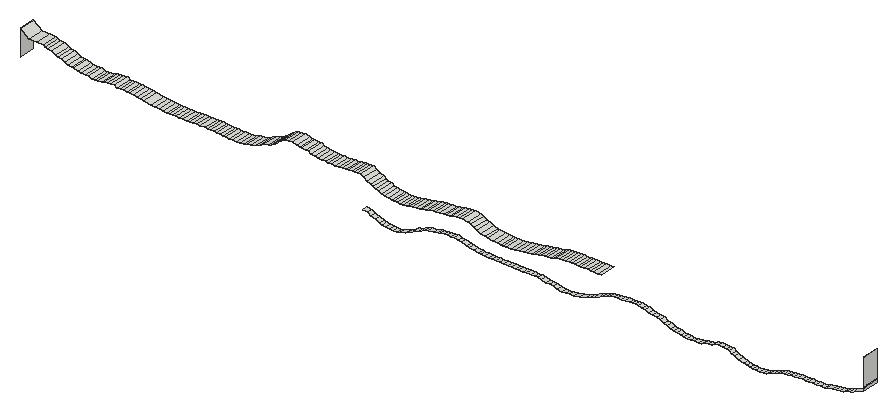
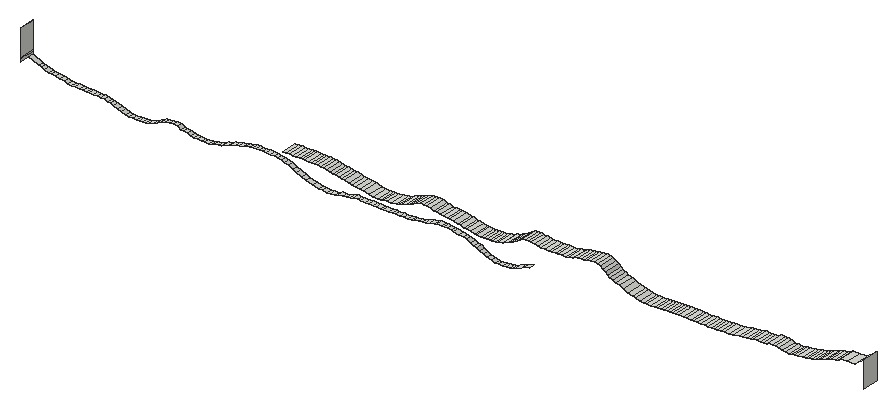
# SketchUp Ruby script. Lengths in inches.
U = 1.inch
M = Sketchup.active_model
def pt(a) = Geom::Point3d.new(a.map { |v| v * U })
def face(e, loops, mat)
  f = e.add_face(loops[0].map { |a| pt(a) })
  loops[1..].each { |l| e.add_face(l.map { |a| pt(a) }).erase! }
  f.material = f.back_material = mat if mat
  f
end
# faces: each face lists its corners as indices into pts; further lists are holes
def faces(e, pts, list, mat = nil) = list.each { |f| face(e, (f[0].is_a?(Array) ? f : [f]).map { |l| l.map { |i| pts[i] } }, mat) }
# xy, xz, yz: faces in a plane at the given z, y or x. An outline is a flat list of corners, or four numbers for a rectangle; further outlines are holes
def ring(l) = l.size == 4 ? [[l[0], l[1]], [l[2], l[1]], [l[2], l[3]], [l[0], l[3]]] : l.each_slice(2).to_a
def flat(e, list, mat, &to3) = list.each { |f| face(e, (f[0].is_a?(Array) ? f : [f]).map { |l| ring(l).map { |u, v| to3.(u, v) } }, mat) }
def xy(e, z, list, mat = nil) = flat(e, list, mat) { |x, y| [x, y, z] }
def xz(e, y, list, mat = nil) = flat(e, list, mat) { |x, z| [x, y, z] }
def yz(e, x, list, mat = nil) = flat(e, list, mat) { |y, z| [x, y, z] }
def lines(e, pts, list) = list.each { |a, b| e.add_line(pt(pts[a]), pt(pts[b])) }
# prism: a flat outline (further loops are holes) pulled along v
def prism(e, loops, v, mat = nil)
  f = face(e, loops, mat); d = Geom::Vector3d.new(v.map { |x| x * U })
  f.pushpull(f.normal.samedirection?(d) ? d.length : -d.length)
end
def box(e, o, s, mat = nil) = prism(e, [[o, [o[0] + s[0], o[1], o[2]], [o[0] + s[0], o[1] + s[1], o[2]], [o[0], o[1] + s[1], o[2]]]], [0, 0, s[2]], mat)
def at(x, y, z, deg = 0) = Geom::Transformation.translation(pt([x, y, z])) * Geom::Transformation.rotation(ORIGIN, Z_AXIS, deg.degrees)
def axes(o, x, y, z) = Geom::Transformation.new([*x, 0, *y, 0, *z, 0, *pt(o).to_a, 1])
def part(name) = M.definitions.add(name)
# library, detail: a bought-in or finely detailed component or shape, given as its bounding box
def library(name, o, s) = part(name).tap { |d| box(d.entities, o, s) }
def detail(e, o, s) = box(e.add_group.entities, o, s)
def put(e, d, t, mat = nil) = e.add_instance(d, t).tap { |i| i.material = mat if mat }
def group(e, t, mat = nil) = e.add_group.tap { |g| g.transformation = t; g.material = mat if mat }.entities
root = M.entities
xy(root,238.18,[[3012.28,565.74,3012.96,566.68]])
xy(root,238.62,[[2978.81,565.74,2979.58,566.68],[2979.58,565.74,2980.21,566.68],[2980.21,565.74,2980.97,566.68],[2980.97,565.74,2981.59,566.68],[2981.59,565.74,2982.44,566.68],
  [2982.44,565.74,2983.08,566.68],[2983.08,565.74,2983.7,566.68]])
xy(root,238.625,[[2977.39,565.74,2978.25,566.68]])
xy(root,238.89,[[3033.2,565.74,3033.88,566.68]])
xy(root,238.9,[[3034.64,565.74,3035.26,566.68],[3035.26,565.74,3036.03,566.68]])
xy(root,240.43,[[3001.48,565.74,3002.05,566.68]])
xy(root,241.68,[[2919.53,565.74,2920.12,568.68]])
xy(root,241.75,[[2921.88,565.74,2922.75,568.68],[2922.75,565.74,2923.37,568.68],[2923.37,565.74,2923.88,568.68]])
xy(root,243.05,[[2994.54,565.74,2995.22,568.68]])
xy(root,243.07,[[2992.6875,565.74,2993.27,568.68]])
xy(root,243.09,[[2989.375,565.74,2989.9,568.68],[2989.9,565.74,2990.42,568.68],[2990.42,565.74,2991.08,568.68],[2991.08,565.74,2991.53,568.68]])
yz(root,2889.09,[[565.74,241.52,568.68,246.2]])
yz(root,3043.1,[[565.74,240.89,565.74,241.29,568.68,241.52,568.68,240.89],[565.74,241.29,568.68,241.52,565.74,241.52],[565.74,241.52,565.74,246.27,566.4375,246.36,568.68,246.43,568.68,241.52],[565.74,246.27,565.74,246.43,568.68,246.43,566.4375,246.36]])
p = [[2955.89,565.74,237.11],[2955.89,566.68,237.11],[2956.65,566.68,237.04],[2956.65,565.74,237.04],[2957.34,566.68,237.01],[2957.34,565.74,237.01],
  [2957.95,566.68,236.98],[2957.95,565.74,236.98],[2958.63,566.68,237.22],[2958.63,565.74,237.22],[2955.2,565.74,237.2],[2955.2,566.68,237.2],
  [2954.67,565.74,237.33],[2954.67,566.68,237.33],[2959.48,566.68,237.43],[2959.48,565.74,237.43],[2954,565.74,237.68],[2954,566.68,237.68],
  [2960.1,566.68,237.74],[2960.1,565.74,237.74],[3022.93,565.74,237.45],[3022.93,566.68,237.45],[3023.5,566.68,237.42],[3023.5,565.74,237.42],
  [3024.23,566.68,237.4],[3024.23,565.74,237.4],[3024.91,566.68,237.47],[3024.91,565.74,237.47],[3021.74,565.74,237.59],[3021.74,566.68,237.59],
  [3022.34,566.68,237.51],[3022.34,565.74,237.51],[3025.51,566.68,237.5625],[3025.51,565.74,237.5625],[3021.2,565.74,237.71],[3021.2,566.68,237.71],
  [3026.2,566.68,237.84],[3026.2,565.74,237.84],[2953.0625,565.74,237.96],[2953.0625,566.68,237.96],[2960.8,566.68,238.02],[2960.8,565.74,238.02],
  [2987.94,565.74,237.79],[2987.94,566.68,237.79],[2988.65,566.68,237.74],[2988.65,565.74,237.74],[2989.52,566.68,237.87],[2989.52,565.74,237.87],
  [3020.37,565.74,238],[3020.37,566.68,238],[2987.17,565.74,237.86],[2987.17,566.68,237.86],[3026.88,566.68,238.08],[3026.88,565.74,238.08],
  [2986.54,565.74,238.15],[2986.54,566.68,238.15],[2990.17,566.68,237.88],[2990.17,565.74,237.88],[2991.29,566.68,238.14],[2991.29,565.74,238.14],
  [2952.5,565.74,238.28],[2952.5,566.68,238.28],[2961.24,566.68,238.375],[2961.24,565.74,238.375],[3019.66,565.74,238.33],[3019.66,566.68,238.33],
  [2985.77,565.74,238.19],[2985.77,566.68,238.19],[2992.51,566.68,238.46],[2992.51,565.74,238.46],[3010.26,565.74,238.19],[3010.26,566.68,238.19],
  [3011.08,566.68,238.15],[3011.08,565.74,238.15],[3011.61,566.68,238.11],[3011.61,565.74,238.11],[3012.28,566.68,238.18],[3012.28,565.74,238.18],
  [3027.57,566.68,238.33],[3027.57,565.74,238.33],[2985.15,565.74,238.25],[2985.15,566.68,238.25],[3009.6875,565.74,238.26],[3009.6875,566.68,238.26],
  [3012.96,565.74,238.18],[3012.96,566.68,238.18],[3013.64,566.68,238.27],[3013.64,565.74,238.27],[2951.72,565.74,238.43],[2951.72,566.68,238.43],
  [2984.39,565.74,238.45],[2984.39,566.68,238.45],[3009.12,565.74,238.48],[3009.12,566.68,238.48],[3014.16,566.68,238.55],[3014.16,565.74,238.55],
  [3019.11,565.74,238.57],[3019.11,566.68,238.57],[3028.1,566.68,238.51],[3028.1,565.74,238.51],[2961.8,566.68,238.51],[2961.8,565.74,238.51],
  [2962.4375,566.68,238.76],[2962.4375,565.74,238.76],[2983.7,565.74,238.62],[2983.7,566.68,238.62],[2993.26,566.68,238.72],[2993.26,565.74,238.72],
  [3008.46,565.74,238.56],[3008.46,566.68,238.56],[3014.82,566.68,238.61],[3014.82,565.74,238.61],[3028.67,566.68,238.6],[3028.67,565.74,238.6],
  [2974.63,565.74,238.66],[2974.63,566.68,238.66],[2975.3,566.68,238.65],[2975.3,565.74,238.65],[2976.08,566.68,238.64],[2976.08,565.74,238.64],
  [2976.7,566.68,238.63],[2976.7,565.74,238.63],[2977.39,566.68,238.625],[2977.39,565.74,238.625],[2978.25,565.74,238.625],[2978.25,566.68,238.625],
  [2978.81,566.68,238.62],[2978.81,565.74,238.62],[3007.89,565.74,238.67],[3007.89,566.68,238.67],[3015.41,566.68,238.66],[3015.41,565.74,238.66],
  [3018.61,565.74,238.86],[3018.61,566.68,238.86],[3029.33,566.68,238.74],[3029.33,565.74,238.74],[2972.79,565.74,238.78],[2972.79,566.68,238.78],
  [2973.27,566.68,238.73],[2973.27,565.74,238.73],[2973.94,566.68,238.6875],[2973.94,565.74,238.6875],[2994.14,566.68,239.08],[2994.14,565.74,239.08],
  [3007.37,565.74,239.01],[3007.37,566.68,239.01],[3015.98,566.68,239.04],[3015.98,565.74,239.04],[3029.91,566.68,238.8],[3029.91,565.74,238.8],
  [2963.08,566.68,239.12],[2963.08,565.74,239.12],[2971.91,565.74,238.93],[2971.91,566.68,238.93],[3030.48,566.68,238.83],[3030.48,565.74,238.83],
  [3031.22,566.68,238.86],[3031.22,565.74,238.86],[2971.14,565.74,239.07],[2971.14,566.68,239.07],[3018.09,565.74,238.96],[3018.09,566.68,238.96],
  [3031.98,566.68,238.875],[3031.98,565.74,238.875],[3032.52,566.68,238.88],[3032.52,565.74,238.88],[3033.2,566.68,238.89],[3033.2,565.74,238.89],
  [3033.88,565.74,238.89],[3033.88,566.68,238.89],[3034.64,566.68,238.9],[3034.64,565.74,238.9],[3036.03,565.74,238.9],[3036.03,566.68,238.9],
  [3036.66,566.68,239.15],[3036.66,565.74,239.15],[3006.6875,565.74,239.18],[3006.6875,566.68,239.18],[3016.72,566.68,239.125],[3016.72,565.74,239.125],
  [3017.4,566.68,239.02],[3017.4,565.74,239.02],[2963.66,566.68,239.22],[2963.66,565.74,239.22],[2970.59,565.74,239.16],[2970.59,566.68,239.16],
  [2994.93,566.68,239.375],[2994.93,565.74,239.375],[2964.66,566.68,239.31],[2964.66,565.74,239.31],[2969.74,565.74,239.44],[2969.74,566.68,239.44],
  [3006.0625,565.74,239.5],[3006.0625,566.68,239.5],[3037.43,566.68,239.28],[3037.43,565.74,239.28],[2965.47,566.68,239.54],[2965.47,565.74,239.54],
  [3038.23,566.68,239.42],[3038.23,565.74,239.42],[2969.07,565.74,239.56],[2969.07,566.68,239.56],[2995.67,566.68,239.75],[2995.67,565.74,239.75],
  [3038.95,566.68,239.49],[3038.95,565.74,239.49],[2965.96,566.68,239.6],[2965.96,565.74,239.6],[3005.3,565.74,239.65],[3005.3,566.68,239.65],
  [3039.5,566.68,239.53],[3039.5,565.74,239.53],[3040.1875,566.68,239.81],[3040.1875,565.74,239.81],[2966.58,566.68,239.65],[2966.58,565.74,239.65],
  [2967.17,566.68,239.69],[2967.17,565.74,239.69],[2968.46,565.74,239.72],[2968.46,566.68,239.72],[2967.73,566.68,239.7],[2967.73,565.74,239.7],
  [2996.32,566.68,239.97],[2996.32,565.74,239.97],[3004.6875,565.74,239.8],[3004.6875,566.68,239.8],[3003.93,565.74,239.96],[3003.93,566.68,239.96],
  [3040.71,566.68,239.96],[3040.71,565.74,239.96],[2996.94,566.68,240.17],[2996.94,565.74,240.17],[3003.28,565.74,240.23],[3003.28,566.68,240.23],
  [3041.27,566.68,240.1],[3041.27,565.74,240.1],[3043.1,566.68,240.89],[3043.1,565.74,240.89],[2997.62,566.68,240.27],[2997.62,565.74,240.27],
  [3002.7,565.74,240.27],[3002.7,566.68,240.27],[2998.3,566.68,240.33],[2998.3,565.74,240.33],[2998.99,566.68,240.37],[2998.99,565.74,240.37],
  [3002.05,565.74,240.43],[3002.05,566.68,240.43],[2999.68,566.68,240.4],[2999.68,565.74,240.4],[3000.375,566.68,240.41],[3000.375,565.74,240.41],
  [3000.9,566.68,240.42],[3000.9,565.74,240.42],[3001.48,566.68,240.43],[3001.48,565.74,240.43],[2925.51,568.68,241.57],[2926.05,568.68,241.53],
  [2926.05,565.74,241.53],[2925.51,565.74,241.57],[2926.67,568.68,241.51],[2926.67,565.74,241.51],[2927.22,568.68,241.49],[2927.22,565.74,241.49],
  [2927.92,568.68,241.48],[2927.92,565.74,241.48],[2928.58,568.68,241.47],[2928.58,565.74,241.47],[2929.15,568.68,241.46],[2929.15,565.74,241.46],
  [2929.86,568.68,241.6],[2929.86,565.74,241.6],[2976.23,568.68,241.56],[2976.83,568.68,241.51],[2976.83,565.74,241.51],[2976.23,565.74,241.56],
  [2977.28,568.68,241.48],[2977.28,565.74,241.48],[2977.8,568.68,241.46],[2977.8,565.74,241.46],[2978.67,568.68,241.51],[2978.67,565.74,241.51],
  [2979.39,568.68,241.59],[2979.39,565.74,241.59],[2924.9,568.68,241.66],[2924.9,565.74,241.66],[2930.59,568.68,241.85],[2930.59,565.74,241.85],
  [2974.41,568.68,241.78],[2975.46,568.68,241.63],[2975.46,565.74,241.63],[2974.41,565.74,241.78],[2980.33,568.68,241.82],[2980.33,565.74,241.82],
  [2915.87,568.68,241.75],[2916.32,568.68,241.74],[2916.32,565.74,241.74],[2915.87,565.74,241.75],[2916.87,568.68,241.72],[2916.87,565.74,241.72],
  [2917.5,568.68,241.71],[2917.5,565.74,241.71],[2918.13,568.68,241.7],[2918.13,565.74,241.7],[2918.86,568.68,241.69],[2918.86,565.74,241.69],
  [2919.53,568.68,241.68],[2919.53,565.74,241.68],[2920.12,568.68,241.68],[2920.61,568.68,241.67],[2920.61,565.74,241.67],[2920.12,565.74,241.68],
  [2921.3125,568.68,241.74],[2921.3125,565.74,241.74],[2921.88,568.68,241.75],[2921.88,565.74,241.75],[2923.88,568.68,241.75],[2924.37,568.68,241.67],
  [2924.37,565.74,241.67],[2923.88,565.74,241.75],[2913.68,568.68,241.89],[2914.5,568.68,241.83],[2914.5,565.74,241.83],[2913.68,565.74,241.89],
  [2915.1,568.68,241.78],[2915.1,565.74,241.78],[2931.26,568.68,241.91],[2931.26,565.74,241.91],[2956.89,568.68,241.89],[2957.35,568.68,241.85],
  [2957.35,565.74,241.85],[2956.89,565.74,241.89],[2957.87,568.68,241.8125],[2957.87,565.74,241.8125],[2958.38,568.68,241.79],[2958.38,565.74,241.79],
  [2958.96,568.68,241.78],[2958.96,565.74,241.78],[2959.63,568.68,241.91],[2959.63,565.74,241.91],[2973.92,568.68,241.89],[2973.92,565.74,241.89],
  [2981.11,568.68,241.87],[2981.11,565.74,241.87],[2912.91,568.68,241.96],[2912.91,565.74,241.96],[2932.16,568.68,242.1],[2932.16,565.74,242.1],
  [2956.33,568.68,241.96],[2956.33,565.74,241.96],[2960.1,568.68,241.93],[2960.1,565.74,241.93],[2960.77,568.68,242.09],[2960.77,565.74,242.09],
  [2973.28,568.68,242.14],[2973.28,565.74,242.14],[2981.875,568.68,241.98],[2981.875,565.74,241.98],[2911.74,568.68,242.24],[2911.74,565.74,242.24],
  [2955.65,568.68,242.11],[2955.65,565.74,242.11],[2982.49,568.68,242.02],[2982.49,565.74,242.02],[2983.14,568.68,242.19],[2983.14,565.74,242.19],
  [2932.93,568.68,242.46],[2932.93,565.74,242.46],[2955.05,568.68,242.21],[2955.05,565.74,242.21],[2961.54,568.68,242.2],[2961.54,565.74,242.2],
  [2972.52,568.68,242.39],[2972.52,565.74,242.39],[2911.07,568.68,242.34],[2911.07,565.74,242.34],[2954.54,568.68,242.51],[2954.54,565.74,242.51],
  [2962.04,568.68,242.24],[2962.04,565.74,242.24],[2962.65,568.68,242.42],[2962.65,565.74,242.42],[2983.84,568.68,242.38],[2983.84,565.74,242.38],
  [2910.41,568.68,242.38],[2910.41,565.74,242.38],[2909.75,568.68,242.48],[2909.75,565.74,242.48],[2963.2,568.68,242.47],[2963.2,565.74,242.47],
  [2971.9,568.68,242.65],[2971.9,565.74,242.65],[2984.33,568.68,242.4375],[2984.33,565.74,242.4375],[2984.85,568.68,242.48],[2984.85,565.74,242.48],
  [2901.57,568.68,242.68],[2902.24,568.68,242.51],[2902.24,565.74,242.51],[2901.57,565.74,242.68],[2902.76,568.68,242.46],[2902.76,565.74,242.46],
  [2903.3,568.68,242.58],[2903.3,565.74,242.58],[2909.11,568.68,242.57],[2909.11,565.74,242.57],[2933.63,568.68,242.78],[2933.63,565.74,242.78],
  [2953.95,568.68,242.68],[2953.95,565.74,242.68],[2963.95,568.68,242.71],[2963.95,565.74,242.71],[2985.51,568.68,242.58],[2985.51,565.74,242.58],
  [2903.93,568.68,242.57],[2903.93,565.74,242.57],[2904.56,568.68,242.81],[2904.56,565.74,242.81],[2906.33,568.68,242.92],[2906.76,568.68,242.625],
  [2906.76,565.74,242.625],[2906.33,565.74,242.92],[2907.37,568.68,242.65],[2907.37,565.74,242.65],[2907.92,568.68,242.62],[2907.92,565.74,242.62],
  [2908.55,568.68,242.58],[2908.55,565.74,242.58],[2971.35,568.68,242.9375],[2971.35,565.74,242.9375],[2986.04,568.68,242.61],[2986.04,565.74,242.61],
  [2986.625,568.68,242.77],[2986.625,565.74,242.77],[2900.22,568.68,242.78],[2901.03,568.68,242.73],[2901.03,565.74,242.73],[2900.22,565.74,242.78],
  [2953.45,568.68,242.875],[2953.45,565.74,242.875],[2964.59,568.68,242.78],[2964.59,565.74,242.78],[2898.92,568.68,243.06],[2899.64,568.68,242.85],
  [2899.64,565.74,242.85],[2898.92,565.74,243.06],[2905.13,568.68,242.86],[2905.13,565.74,242.86],[2934.4,568.68,242.97],[2934.4,565.74,242.97],
  [2965.07,568.68,242.82],[2965.07,565.74,242.82],[2965.76,568.68,242.85],[2965.76,565.74,242.85],[2987.08,568.68,242.95],[2987.08,565.74,242.95],
  [2905.69,568.68,242.89],[2905.69,565.74,242.89],[2953.06,568.68,243.09],[2953.06,565.74,243.09],[2966.46,568.68,242.87],[2966.46,565.74,242.87],
  [2967.01,568.68,243.02],[2967.01,565.74,243.02],[2970.78,568.68,243.14],[2970.78,565.74,243.14],[2934.93,568.68,243.23],[2934.93,565.74,243.23],
  [2967.63,568.68,243.05],[2967.63,565.74,243.05],[2987.64,568.68,243.01],[2987.64,565.74,243.01],[2988.15,568.68,243.05],[2988.15,565.74,243.05],
  [2988.72,568.68,243.08],[2988.72,565.74,243.08],[2897.85,568.68,243.3],[2898.4375,568.68,243.14],[2898.4375,565.74,243.14],[2897.85,565.74,243.3],
  [2952.45,568.68,243.43],[2952.45,565.74,243.43],[2968.18,568.68,243.29],[2968.18,565.74,243.29],[2970.01,568.68,243.42],[2970.01,565.74,243.42],
  [2989.375,568.68,243.09],[2989.375,565.74,243.09],[2991.53,568.68,243.09],[2992.1,568.68,243.08],[2992.1,565.74,243.08],[2991.53,565.74,243.09],
  [2992.6875,568.68,243.07],[2992.6875,565.74,243.07],[2993.27,568.68,243.07],[2993.93,568.68,243.0625],[2993.93,565.74,243.0625],[2993.27,565.74,243.07],
  [2994.54,568.68,243.05],[2994.54,565.74,243.05],[2935.33,568.68,243.48],[2935.33,565.74,243.48],[2897.21,568.68,243.48],[2897.21,565.74,243.48],
  [2968.86,568.68,243.35],[2968.86,565.74,243.35],[2951.91,568.68,243.8],[2951.91,565.74,243.8],[2969.41,568.68,243.39],[2969.41,565.74,243.39],
  [2896.69,568.68,243.79],[2896.69,565.74,243.79],[2935.85,568.68,243.72],[2935.85,565.74,243.72],[2936.1875,568.68,244.12],[2936.1875,565.74,244.12],
  [2896.03,568.68,243.95],[2896.03,565.74,243.95],[2951.31,568.68,244.18],[2951.31,565.74,244.18],[2895.51,568.68,244.11],[2895.51,565.74,244.11],
  [2944.13,568.68,243.99],[2944.85,568.68,243.95],[2944.85,565.74,243.95],[2944.13,565.74,243.99],[2945.35,568.68,243.93],[2945.35,565.74,243.93],
  [2946.04,568.68,243.91],[2946.04,565.74,243.91],[2946.61,568.68,243.89],[2946.61,565.74,243.89],[2947.31,568.68,243.88],[2947.31,565.74,243.88],
  [2947.96,568.68,243.94],[2947.96,565.74,243.94],[2948.6,568.68,243.95],[2948.6,565.74,243.95],[2949.16,568.68,244.1],[2949.16,565.74,244.1],
  [2942.95,568.68,244.11],[2943.51,568.68,244.04],[2943.51,565.74,244.04],[2942.95,565.74,244.11],[2894.84,568.68,244.41],[2894.84,565.74,244.41],
  [2936.66,568.68,244.39],[2936.66,565.74,244.39],[2942.2,568.68,244.25],[2942.2,565.74,244.25],[2949.79,568.68,244.13],[2949.79,565.74,244.13],
  [2950.27,568.68,244.15],[2950.27,565.74,244.15],[2950.79,568.68,244.17],[2950.79,565.74,244.17],[2941.74,568.68,244.51],[2941.74,565.74,244.51],
  [2894.08,568.68,244.54],[2894.08,565.74,244.54],[2937.14,568.68,244.73],[2937.14,565.74,244.73],[2893.52,568.68,244.61],[2893.52,565.74,244.61],
  [2940.59,568.68,244.67],[2941.2,568.68,244.55],[2941.2,565.74,244.55],[2940.59,565.74,244.67],[2893.3,568.68,244.92],[2893.3,565.74,244.92],
  [2937.625,568.68,244.87],[2937.625,565.74,244.87],[2939.54,568.68,244.81],[2940.11,568.68,244.7],[2940.11,565.74,244.7],[2939.54,565.74,244.81],
  [2938.89,568.68,245.01],[2938.89,565.74,245.01],[2890.66,568.68,244.96],[2892.05,568.68,244.9375],[2892.05,565.74,244.9375],[2890.66,565.74,244.96],
  [2938.21,568.68,244.95],[2938.21,565.74,244.95],[2889.09,568.68,246.2],[2889.09,565.74,246.2]]
faces(root,p,[[0,1,2,3],[3,2,4,5],[5,4,6,7],[7,6,8,9],[10,11,1,0],[12,13,11,10],[9,8,14,15],[16,17,13,12],
  [15,14,18,19],[20,21,22,23],[23,22,24,25],[25,24,26,27],[28,29,30,31],[31,30,21,20],[27,26,32,33],[34,35,29,28],
  [33,32,36,37],[38,39,17,16],[19,18,40,41],[42,43,44,45],[45,44,46,47],[48,49,35,34],[50,51,43,42],[37,36,52,53],
  [54,55,51,50],[47,46,56,57],[57,56,58,59],[60,61,39,38],[41,40,62,63],[64,65,49,48],[66,67,55,54],[59,58,68,69],
  [70,71,72,73],[73,72,74,75],[75,74,76,77],[53,52,78,79],[80,81,67,66],[82,83,71,70],[84,85,86,87],[88,89,61,60],
  [90,91,81,80],[92,93,83,82],[87,86,94,95],[96,97,65,64],[79,78,98,99],[63,62,100,101],[101,100,102,103],[104,105,91,90],
  [69,68,106,107],[108,109,93,92],[95,94,110,111],[99,98,112,113],[114,115,116,117],[117,116,118,119],[119,118,120,121],[121,120,122,123],
  [124,125,126,127],[128,129,109,108],[111,110,130,131],[132,133,97,96],[113,112,134,135],[136,137,138,139],[139,138,140,141],[141,140,115,114],
  [107,106,142,143],[144,145,129,128],[131,130,146,147],[135,134,148,149],[103,102,150,151],[152,153,137,136],[149,148,154,155],[155,154,156,157],
  [158,159,153,152],[160,161,133,132],[157,156,162,163],[163,162,164,165],[165,164,166,167],[168,169,170,171],[172,173,174,175],[176,177,145,144],
  [147,146,178,179],[179,178,180,181],[181,180,161,160],[151,150,182,183],[184,185,159,158],[143,142,186,187],[183,182,188,189],[190,191,185,184],
  [192,193,177,176],[175,174,194,195],[189,188,196,197],[195,194,198,199],[200,201,191,190],[187,186,202,203],[199,198,204,205],[197,196,206,207],
  [208,209,193,192],[205,204,210,211],[211,210,212,213],[207,206,214,215],[215,214,216,217],[218,219,201,200],[217,216,220,221],[221,220,219,218],
  [203,202,222,223],[224,225,209,208],[226,227,225,224],[213,212,228,229],[223,222,230,231],[232,233,227,226],[229,228,234,235],[235,234,236,237],
  [231,230,238,239],[240,241,233,232],[239,238,242,243],[243,242,244,245],[246,247,241,240],[245,244,248,249],[249,248,250,251],[251,250,252,253],
  [253,252,254,255],[256,257,258,259],[257,260,261,258],[260,262,263,261],[262,264,265,263],[264,266,267,265],[266,268,269,267],[268,270,271,269],
  [272,273,274,275],[273,276,277,274],[276,278,279,277],[278,280,281,279],[280,282,283,281],[284,256,259,285],[270,286,287,271],[288,289,290,291],
  [289,272,275,290],[282,292,293,283],[294,295,296,297],[295,298,299,296],[298,300,301,299],[300,302,303,301],[302,304,305,303],[304,306,307,305],
  [308,309,310,311],[309,312,313,310],[312,314,315,313],[316,317,318,319],[317,284,285,318],[320,321,322,323],[321,324,325,322],[324,294,297,325],
  [286,326,327,287],[328,329,330,331],[329,332,333,330],[332,334,335,333],[334,336,337,335],[336,338,339,337],[340,288,291,341],[292,342,343,293],
  [344,320,323,345],[326,346,347,327],[348,328,331,349],[338,350,351,339],[350,352,353,351],[354,340,341,355],[342,356,357,343],[358,344,345,359],
  [360,348,349,361],[356,362,363,357],[362,364,365,363],[346,366,367,347],[368,360,361,369],[352,370,371,353],[372,354,355,373],[374,358,359,375],
  [376,368,369,377],[370,378,379,371],[378,380,381,379],[364,382,383,365],[384,374,375,385],[386,384,385,387],[380,388,389,381],[390,372,373,391],
  [382,392,393,383],[392,394,395,393],[396,397,398,399],[397,400,401,398],[400,402,403,401],[404,386,387,405],[366,406,407,367],[408,376,377,409],
  [388,410,411,389],[394,412,413,395],[402,414,415,403],[414,416,417,415],[418,419,420,421],[419,422,423,420],[422,424,425,423],[424,426,427,425],
  [426,404,405,427],[428,390,391,429],[412,430,431,413],[430,432,433,431],[434,435,436,437],[435,396,399,436],[438,408,409,439],[410,440,441,411],
  [442,443,444,445],[443,434,437,444],[416,446,447,417],[406,448,449,407],[440,450,451,441],[450,452,453,451],[432,454,455,433],[446,456,457,447],
  [456,418,421,457],[458,438,439,459],[452,460,461,453],[460,462,463,461],[464,428,429,465],[448,466,467,449],[462,468,469,463],[454,470,471,455],
  [470,472,473,471],[472,474,475,473],[476,477,478,479],[477,442,445,478],[480,458,459,481],[468,482,483,469],[484,464,465,485],[474,486,487,475],
  [488,489,490,491],[489,492,493,490],[494,495,496,497],[495,498,499,496],[466,500,501,467],[502,476,479,503],[482,504,505,483],[506,480,481,507],
  [504,508,509,505],[508,484,485,509],[510,502,503,511],[500,512,513,501],[512,514,515,513],[516,510,511,517],[518,506,507,519],[520,516,517,521],
  [522,523,524,525],[523,526,527,524],[526,528,529,527],[528,530,531,529],[530,532,533,531],[532,534,535,533],[534,536,537,535],[536,538,539,537],
  [540,541,542,543],[541,522,525,542],[544,520,521,545],[514,546,547,515],[548,540,543,549],[538,550,551,539],[550,552,553,551],[552,554,555,553],
  [554,518,519,555],[556,548,549,557],[558,544,545,559],[546,560,561,547],[562,558,559,563],[564,565,566,567],[565,556,557,566],[568,562,563,569],
  [560,570,571,561],[572,573,574,575],[573,564,567,574],[576,572,575,577],[578,579,580,581],[579,568,569,580],[570,582,583,571],[582,576,577,583],
  [584,578,581,585]])
